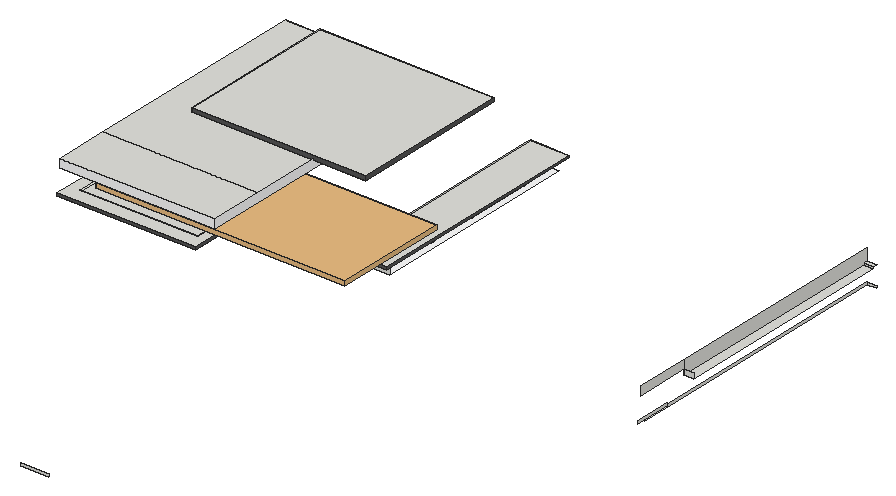
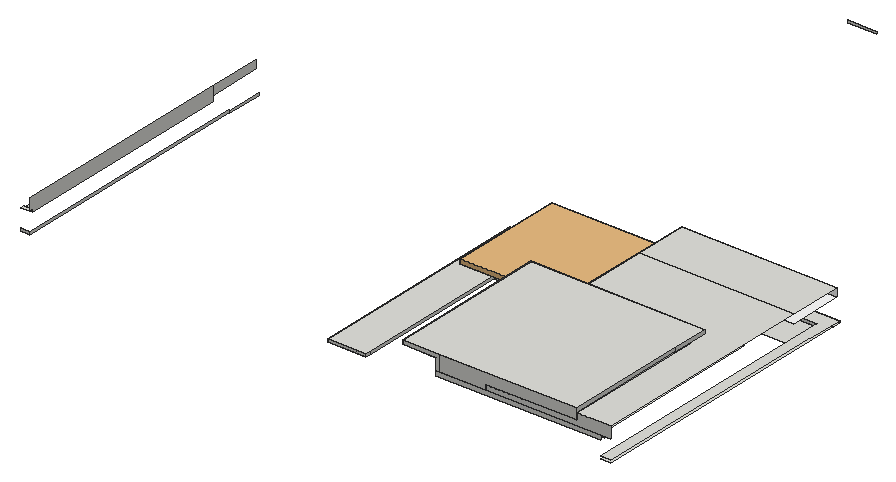
# SketchUp Ruby script. Lengths in inches.
U = 1.inch
M = Sketchup.active_model
def pt(a) = Geom::Point3d.new(a.map { |v| v * U })
def face(e, loops, mat)
  f = e.add_face(loops[0].map { |a| pt(a) })
  loops[1..].each { |l| e.add_face(l.map { |a| pt(a) }).erase! }
  f.material = f.back_material = mat if mat
  f
end
# faces: each face lists its corners as indices into pts; further lists are holes
def faces(e, pts, list, mat = nil) = list.each { |f| face(e, (f[0].is_a?(Array) ? f : [f]).map { |l| l.map { |i| pts[i] } }, mat) }
# xy, xz, yz: faces in a plane at the given z, y or x. An outline is a flat list of corners, or four numbers for a rectangle; further outlines are holes
def ring(l) = l.size == 4 ? [[l[0], l[1]], [l[2], l[1]], [l[2], l[3]], [l[0], l[3]]] : l.each_slice(2).to_a
def flat(e, list, mat, &to3) = list.each { |f| face(e, (f[0].is_a?(Array) ? f : [f]).map { |l| ring(l).map { |u, v| to3.(u, v) } }, mat) }
def xy(e, z, list, mat = nil) = flat(e, list, mat) { |x, y| [x, y, z] }
def xz(e, y, list, mat = nil) = flat(e, list, mat) { |x, z| [x, y, z] }
def yz(e, x, list, mat = nil) = flat(e, list, mat) { |y, z| [x, y, z] }
def lines(e, pts, list) = list.each { |a, b| e.add_line(pt(pts[a]), pt(pts[b])) }
# prism: a flat outline (further loops are holes) pulled along v
def prism(e, loops, v, mat = nil)
  f = face(e, loops, mat); d = Geom::Vector3d.new(v.map { |x| x * U })
  f.pushpull(f.normal.samedirection?(d) ? d.length : -d.length)
end
def box(e, o, s, mat = nil) = prism(e, [[o, [o[0] + s[0], o[1], o[2]], [o[0] + s[0], o[1] + s[1], o[2]], [o[0], o[1] + s[1], o[2]]]], [0, 0, s[2]], mat)
def at(x, y, z, deg = 0) = Geom::Transformation.translation(pt([x, y, z])) * Geom::Transformation.rotation(ORIGIN, Z_AXIS, deg.degrees)
def axes(o, x, y, z) = Geom::Transformation.new([*x, 0, *y, 0, *z, 0, *pt(o).to_a, 1])
def part(name) = M.definitions.add(name)
# library, detail: a bought-in or finely detailed component or shape, given as its bounding box
def library(name, o, s) = part(name).tap { |d| box(d.entities, o, s) }
def detail(e, o, s) = box(e.add_group.entities, o, s)
def put(e, d, t, mat = nil) = e.add_instance(d, t).tap { |i| i.material = mat if mat }
def group(e, t, mat = nil) = e.add_group.tap { |g| g.transformation = t; g.material = mat if mat }.entities
root = M.entities
M.materials.add("[Color M00]").color = [255, 255, 255]
M.materials.add("[Color M06]").color = [86, 86, 86]
c1 = library("Mesh Light\#4",[-0.5,-0.5,-0.1],[1,1,0.2])
c2 = part("Group\#24")
xy(c2.entities,0,[[203.13,95.41,201.58,95.62,200.13,96.22,198.89,97.17,197.9375,98.41,197.34,99.86,197.13,101.41,197.34,102.96,197.9375,104.41,198.89,105.65,200.13,106.61,201.58,107.21,203.13,107.41,204.6875,107.21,206.13,106.61,207.375,105.65,208.33,104.41,208.93,102.96,209.13,101.41,208.93,99.86,208.33,98.41,207.375,97.17,206.13,96.22,204.6875,95.62],[281.57,95.41,280.02,95.62,278.57,96.22,277.33,97.17,276.375,98.41,275.77,99.86,275.57,101.41,275.77,102.96,276.375,104.41,277.33,105.65,278.57,106.61,280.02,107.21,281.57,107.41,283.125,107.21,284.57,106.61,285.8125,105.65,286.77,104.41,287.37,102.96,287.57,101.41,287.37,99.86,286.77,98.41,285.8125,97.17,284.57,96.22,283.125,95.62],[350.95,95.41,349.39,95.62,347.95,96.22,346.7,97.17,345.75,98.41,345.15,99.86,344.95,101.41,345.15,102.96,345.75,104.41,346.7,105.65,347.95,106.61,349.39,107.21,350.95,107.41,352.5,107.21,353.95,106.61,355.1875,105.65,356.14,104.41,356.74,102.96,356.95,101.41,356.74,99.86,356.14,98.41,355.1875,97.17,353.95,96.22,352.5,95.62],[376,162.85,374.44,163.05,373,163.65,371.75,164.6,370.8,165.85,370.2,167.29,370,168.85,370.2,170.4,370.8,171.85,371.75,173.09,373,174.04,374.44,174.64,376,174.85,377.55,174.64,379,174.04,380.24,173.09,381.19,171.85,381.79,170.4,382,168.85,381.79,167.29,381.19,165.85,380.24,164.6,379,163.65,377.55,163.05]],"[Color M00]")
xy(c2.entities,33.4375,[[6,0,4.45,0.2,3,0.8,1.76,1.76,0.8,3,0.2,4.45,0,6,0.2,7.55,0.8,9,1.76,10.24,3,11.2,4.45,11.8,6,12,7.55,11.8,9,11.2,10.24,10.24,11.2,9,11.8,7.55,12,6,11.8,4.45,11.2,3,10.24,1.76,9,0.8,7.55,0.2],[83.125,0,81.57,0.2,80.125,0.8,78.88,1.76,77.93,3,77.33,4.45,77.125,6,77.33,7.55,77.93,9,78.88,10.24,80.125,11.2,81.57,11.8,83.125,12,84.68,11.8,86.125,11.2,87.37,10.24,88.32,9,88.92,7.55,89.125,6,88.92,4.45,88.32,3,87.37,1.76,86.125,0.8,84.68,0.2],[166.6875,0,165.13,0.2,163.6875,0.8,162.44,1.76,161.49,3,160.89,4.45,160.6875,6,160.89,7.55,161.49,9,162.44,10.24,163.6875,11.2,165.13,11.8,166.6875,12,168.24,11.8,169.6875,11.2,170.93,10.24,171.88,9,172.48,7.55,172.6875,6,172.48,4.45,171.88,3,170.93,1.76,169.6875,0.8,168.24,0.2],[166.6875,88.9375,165.13,89.14,163.6875,89.74,162.44,90.69,161.49,91.9375,160.89,93.38,160.6875,94.9375,160.89,96.49,161.49,97.9375,162.44,99.18,163.6875,100.13,165.13,100.73,166.6875,100.9375,168.24,100.73,169.6875,100.13,170.93,99.18,171.88,97.9375,172.48,96.49,172.6875,94.9375,172.48,93.38,171.88,91.9375,170.93,90.69,169.6875,89.74,168.24,89.14]],"[Color M00]")
put(c2.entities,c1,axes([191,87.42,16.72],[382.99758,0,0],[0,175.84579,0],[0,0,34.4375]))
c3 = library("Group\#23",[-0.5,-0.5,-0.1],[13,110.375,0.2])
xy(root,270.375,[[2063.54,1581.1,2275.98,1592.1],[2064.92,1592.1,2064.92,2018.36,2079.65,2018.36,2079.65,1604.38,2260.47,1604.38,2260.47,1703.22,2269.48,1703.22,2269.48,1592.1],[2269.48,1592.1,2275.98,1636.04],[2956.13,1592.1,2957.51,1636.04],[2079.65,1604.38,2260.47,1604.38,2260.47,1703.22,2256.86,1703.22,2256.86,1659.57,2079.65,1659.57],
  [2269.48,1636.04,2275.98,1728.29],[2256.86,1703.22,2269.48,1773.67]])
xy(root,274.0625,[[2063.54,1581.1,2275.98,1581.1,2275.98,1673.72,2269.48,1673.72,2269.48,1703.22,2260.47,1703.22,2260.47,1604.38,2079.65,1604.38,2079.65,2018.36,2064.92,2018.36,2064.92,1636.04,2063.54,1636.04],[2269.48,1673.72,2275.98,1728.29]])
xy(root,274.0625,[[[2275.98,1673.72,2275.98,1728.29,2459.67,1728.29,2459.67,1998.71,2500.29,1998.71,2500.29,1673.72],[2311.19,1695.77,2312.75,1695.97,2314.19,1696.57,2315.4375,1697.52,2316.39,1698.77,2316.99,1700.21,2317.19,1701.77,2316.99,1703.32,2316.39,1704.77,2315.4375,1706.01,2314.19,1706.96,2312.75,1707.5625,2311.19,1707.77,2309.64,1707.5625,2308.19,1706.96,2306.95,1706.01,2306,1704.77,2305.4,1703.32,2305.19,1701.77,2305.4,1700.21,2306,1698.77,2306.95,1697.52,2308.19,1696.57,2309.64,1695.97],[2389.63,1695.77,2391.19,1695.97,2392.63,1696.57,2393.875,1697.52,2394.83,1698.77,2395.43,1700.21,2395.63,1701.77,2395.43,1703.32,2394.83,1704.77,2393.875,1706.01,2392.63,1706.96,2391.19,1707.5625,2389.63,1707.77,2388.08,1707.5625,2386.63,1706.96,2385.39,1706.01,2384.4375,1704.77,2383.84,1703.32,2383.63,1701.77,2383.84,1700.21,2384.4375,1698.77,2385.39,1697.52,2386.63,1696.57,2388.08,1695.97],[2459.01,1695.77,2460.56,1695.97,2462.01,1696.57,2463.25,1697.52,2464.2,1698.77,2464.8,1700.21,2465.01,1701.77,2464.8,1703.32,2464.2,1704.77,2463.25,1706.01,2462.01,1706.96,2460.56,1707.5625,2459.01,1707.77,2457.45,1707.5625,2456.01,1706.96,2454.76,1706.01,2453.8125,1704.77,2453.21,1703.32,2453.01,1701.77,2453.21,1700.21,2453.8125,1698.77,2454.76,1697.52,2456.01,1696.57,2457.45,1695.97],[2484.06,1941.01,2485.61,1941.22,2487.06,1941.82,2488.3,1942.77,2489.26,1944.01,2489.86,1945.46,2490.06,1947.01,2489.86,1948.56,2489.26,1950.01,2488.3,1951.25,2487.06,1952.21,2485.61,1952.81,2484.06,1953.01,2482.51,1952.81,2481.06,1952.21,2479.82,1951.25,2478.86,1950.01,2478.26,1948.56,2478.06,1947.01,2478.26,1945.46,2478.86,1944.01,2479.82,1942.77,2481.06,1941.82,2482.51,1941.22],[2484.06,1763.2,2485.61,1763.4,2487.06,1764,2488.3,1764.96,2489.26,1766.2,2489.86,1767.65,2490.06,1769.2,2489.86,1770.75,2489.26,1772.2,2488.3,1773.44,2487.06,1774.4,2485.61,1774.99,2484.06,1775.2,2482.51,1774.99,2481.06,1774.4,2479.82,1773.44,2478.86,1772.2,2478.26,1770.75,2478.06,1769.2,2478.26,1767.65,2478.86,1766.2,2479.82,1764.96,2481.06,1764,2482.51,1763.4],[2484.06,1843.64,2485.61,1843.84,2487.06,1844.44,2488.3,1845.39,2489.26,1846.64,2489.86,1848.08,2490.06,1849.64,2489.86,1851.19,2489.26,1852.64,2488.3,1853.88,2487.06,1854.83,2485.61,1855.43,2484.06,1855.64,2482.51,1855.43,2481.06,1854.83,2479.82,1853.88,2478.86,1852.64,2478.26,1851.19,2478.06,1849.64,2478.26,1848.08,2478.86,1846.64,2479.82,1845.39,2481.06,1844.44,2482.51,1843.84]]],"[Color M00]")
xy(root,283.9375,[[2269.48,1667.47,2500.29,1673.72],[2269.48,1673.72,2269.48,1773.67,2440.84,1773.67,2440.84,2018.36,2500.29,2018.36,2500.29,1673.72]])
xy(root,287.375,[[2269.48,1667.47,2500.29,1667.47,2500.29,2018.36,2440.84,2018.36,2440.84,1773.67,2269.48,1773.67]])
xy(root,295.8125,[[2089.96,1730.8,2089.96,2011.98,2256.86,2011.98,2256.86,1851.54,2247.33,1851.54,2247.33,1730.8],[2256.86,1851.54,2327.29,2011.98]])
xy(root,299.625,[[2957.51,1667.53,2972.24,2011.98]])
xy(root,302.5625,[[2079.65,2011.98,2256.86,2018.36],[2256.86,2011.98,2327.29,2018.36],[2957.51,2011.98,2972.24,2018.36]])
xy(root,307.5,[[[2064.92,1584.22,2064.92,1667.53,2079.65,1667.53,2079.65,1636.22,2256.86,1636.22,2256.86,1829.17,2303.29,1829.17,2303.29,1584.22],[2274.75,1689.29,2276.3,1689.5,2277.75,1690.09,2278.99,1691.05,2279.95,1692.29,2280.54,1693.74,2280.75,1695.29,2280.54,1696.84,2279.95,1698.29,2278.99,1699.53,2277.75,1700.49,2276.3,1701.09,2274.75,1701.29,2273.2,1701.09,2271.75,1700.49,2270.51,1699.53,2269.55,1698.29,2268.95,1696.84,2268.75,1695.29,2268.95,1693.74,2269.55,1692.29,2270.51,1691.05,2271.75,1690.09,2273.2,1689.5],[2114.0625,1600.35,2115.61,1600.56,2117.0625,1601.16,2118.3,1602.11,2119.26,1603.35,2119.86,1604.8,2120.0625,1606.35,2119.86,1607.91,2119.26,1609.35,2118.3,1610.6,2117.0625,1611.55,2115.61,1612.15,2114.0625,1612.35,2112.51,1612.15,2111.0625,1611.55,2109.82,1610.6,2108.87,1609.35,2108.27,1607.91,2108.0625,1606.35,2108.27,1604.8,2108.87,1603.35,2109.82,1602.11,2111.0625,1601.16,2112.51,1600.56],[2191.1875,1600.35,2192.74,1600.56,2194.1875,1601.16,2195.43,1602.11,2196.38,1603.35,2196.98,1604.8,2197.1875,1606.35,2196.98,1607.91,2196.38,1609.35,2195.43,1610.6,2194.1875,1611.55,2192.74,1612.15,2191.1875,1612.35,2189.63,1612.15,2188.1875,1611.55,2186.94,1610.6,2185.99,1609.35,2185.39,1607.91,2185.1875,1606.35,2185.39,1604.8,2185.99,1603.35,2186.94,1602.11,2188.1875,1601.16,2189.63,1600.56],[2274.75,1600.35,2276.3,1600.56,2277.75,1601.16,2278.99,1602.11,2279.95,1603.35,2280.54,1604.8,2280.75,1606.35,2280.54,1607.91,2279.95,1609.35,2278.99,1610.6,2277.75,1611.55,2276.3,1612.15,2274.75,1612.35,2273.2,1612.15,2271.75,1611.55,2270.51,1610.6,2269.55,1609.35,2268.95,1607.91,2268.75,1606.35,2268.95,1604.8,2269.55,1603.35,2270.51,1602.11,2271.75,1601.16,2273.2,1600.56]]],"[Color M00]")
xy(root,310.3125,[[2117.29,1829.17,2256.86,2018.36]])
xy(root,320.75,[[2064.92,1584.22,2303.29,1667.53],[2064.92,1667.53,2303.29,1667.53,2303.29,1771.54,2117.29,1771.54,2117.29,2018.36,2064.92,2018.36],[2303.29,1771.54,2303.29,1829.17,2333.29,1829.17,2333.29,2018.36,2384.86,2018.36,2384.86,1771.54]])
xy(root,326.5,[[2117.29,1771.54,2384.86,2018.36]])
xz(root,1019,[[2456.54,283.9375,2500.29,287.375]])
xz(root,1581.1,[[2063.54,270.375,2275.98,274.0625]],"[Color M06]")
xz(root,1584.22,[[2064.92,307.5,2303.29,320.75]],"[Color M00]")
xz(root,1604.38,[[2079.65,270.375,2260.47,274.0625]])
xz(root,1636.04,[[2956.13,270.375,2957.51,274.0625]])
xz(root,1667.47,[[2269.48,283.9375,2500.29,287.375]],"[Color M06]")
xz(root,1667.53,[[2957.51,299.625,2972.24,307.5]])
xz(root,1673.72,[[2269.48,274.0625,2500.29,283.9375]])
xz(root,1703.22,[[2260.47,270.375,2269.48,274.0625]])
xz(root,1771.54,[[2117.29,320.75,2384.86,326.5]],"[Color M06]")
xz(root,1773.67,[[2269.48,283.9375,2440.84,287.375]])
xz(root,1829.17,[[2256.86,307.5,2303.29,310.3125]])
xz(root,2011.98,[[2079.65,295.8125,2256.86,302.5625],[2256.86,295.8125,2327.29,302.5625],[2957.51,299.625,2972.24,302.5625]])
xz(root,2018.36,[[2957.51,270.375,2972.24,274.0625],[2440.84,283.9375,2456.54,287.375],[2456.54,283.9375,2500.29,287.375],[2079.65,295.8125,2333.29,302.5625],[2064.92,302.5625,2064.92,320.75,2117.29,320.75,2117.29,310.3125,2256.86,310.3125,2256.86,302.5625],
  [2256.86,302.5625,2256.86,310.3125,2117.29,310.3125,2117.29,326.5,2327.29,326.5,2327.29,302.5625],[2327.29,302.5625,2327.29,326.5,2384.86,326.5,2384.86,320.75,2333.29,320.75,2333.29,302.5625]])
yz(root,2117.29,[[1801.17,310.3125,1829.17,320.75],[1829.17,310.3125,2018.36,320.75],[1771.54,320.75,1829.17,326.5],[1829.17,320.75,2018.36,326.5]])
yz(root,2256.86,[[1829.17,295.8125,2011.98,302.5625],[1829.17,302.5625,2018.36,310.3125]])
yz(root,2260.47,[[1604.38,270.375,1703.22,274.0625]])
yz(root,2269.48,[[1728.29,270.375,1728.29,274.0625,1673.72,274.0625,1673.72,283.9375,1773.67,283.9375,1773.67,270.375],[1703.22,270.375,1728.29,274.0625],[1667.47,283.9375,1773.67,287.375]])
yz(root,2275.98,[[1581.1,270.375,1728.29,274.0625]],"[Color M06]")
yz(root,2303.29,[[1584.22,307.5,1829.17,320.75]],"[Color M00]")
yz(root,2384.86,[[1771.54,320.75,2018.36,326.5]],"[Color M06]")
yz(root,2440.84,[[1773.67,283.9375,2011.98,287.375],[2011.98,283.9375,2018.36,287.375]])
yz(root,2500.29,[[1667.47,283.9375,2018.36,287.375]],"[Color M06]")
yz(root,2956.13,[[1581.1,270.375,1636.04,274.0625]])
yz(root,2957.51,[[1636.04,270.375,2018.36,274.0625],[1667.53,299.625,1667.53,320.75,2018.36,320.75,2018.36,302.5625,2011.98,302.5625,2011.98,299.625],[1584.22,307.5,1667.53,320.75]])
p = [[2311.19,1695.77,274.0625],[2309.64,1695.97,274.0625],[2309.64,1695.97,274.75],[2311.19,1695.77,274.75],[2312.75,1695.97,274.0625],[2312.75,1695.97,274.75],
  [2389.63,1695.77,274.0625],[2388.08,1695.97,274.0625],[2388.08,1695.97,274.75],[2389.63,1695.77,274.75],[2391.19,1695.97,274.0625],[2391.19,1695.97,274.75],
  [2459.01,1695.77,274.0625],[2457.45,1695.97,274.0625],[2457.45,1695.97,274.75],[2459.01,1695.77,274.75],[2460.56,1695.97,274.0625],[2460.56,1695.97,274.75],
  [2308.19,1696.57,274.0625],[2308.19,1696.57,274.75],[2314.19,1696.57,274.0625],[2314.19,1696.57,274.75],[2386.63,1696.57,274.0625],[2386.63,1696.57,274.75],
  [2392.63,1696.57,274.0625],[2392.63,1696.57,274.75],[2456.01,1696.57,274.0625],[2456.01,1696.57,274.75],[2462.01,1696.57,274.0625],[2462.01,1696.57,274.75],
  [2306.95,1697.52,274.0625],[2306.95,1697.52,274.75],[2315.4375,1697.52,274.0625],[2315.4375,1697.52,274.75],[2385.39,1697.52,274.0625],[2385.39,1697.52,274.75],
  [2393.875,1697.52,274.0625],[2393.875,1697.52,274.75],[2454.76,1697.52,274.0625],[2454.76,1697.52,274.75],[2463.25,1697.52,274.0625],[2463.25,1697.52,274.75],
  [2306,1698.77,274.0625],[2306,1698.77,274.75],[2316.39,1698.77,274.0625],[2316.39,1698.77,274.75],[2384.4375,1698.77,274.0625],[2384.4375,1698.77,274.75],
  [2394.83,1698.77,274.0625],[2394.83,1698.77,274.75],[2453.8125,1698.77,274.0625],[2453.8125,1698.77,274.75],[2464.2,1698.77,274.0625],[2464.2,1698.77,274.75],
  [2305.4,1700.21,274.0625],[2305.4,1700.21,274.75],[2316.99,1700.21,274.0625],[2316.99,1700.21,274.75],[2383.84,1700.21,274.0625],[2383.84,1700.21,274.75],
  [2395.43,1700.21,274.0625],[2395.43,1700.21,274.75],[2453.21,1700.21,274.0625],[2453.21,1700.21,274.75],[2464.8,1700.21,274.0625],[2464.8,1700.21,274.75],
  [2305.19,1701.77,274.0625],[2305.19,1701.77,274.75],[2317.19,1701.77,274.0625],[2317.19,1701.77,274.75],[2383.63,1701.77,274.0625],[2383.63,1701.77,274.75],
  [2395.63,1701.77,274.0625],[2395.63,1701.77,274.75],[2453.01,1701.77,274.0625],[2453.01,1701.77,274.75],[2465.01,1701.77,274.0625],[2465.01,1701.77,274.75],
  [2305.4,1703.32,274.0625],[2305.4,1703.32,274.75],[2316.99,1703.32,274.0625],[2316.99,1703.32,274.75],[2383.84,1703.32,274.0625],[2383.84,1703.32,274.75],
  [2395.43,1703.32,274.0625],[2395.43,1703.32,274.75],[2453.21,1703.32,274.0625],[2453.21,1703.32,274.75],[2464.8,1703.32,274.0625],[2464.8,1703.32,274.75],
  [2306,1704.77,274.0625],[2306,1704.77,274.75],[2316.39,1704.77,274.0625],[2316.39,1704.77,274.75],[2384.4375,1704.77,274.0625],[2384.4375,1704.77,274.75],
  [2394.83,1704.77,274.0625],[2394.83,1704.77,274.75],[2453.8125,1704.77,274.0625],[2453.8125,1704.77,274.75],[2464.2,1704.77,274.0625],[2464.2,1704.77,274.75],
  [2306.95,1706.01,274.0625],[2306.95,1706.01,274.75],[2315.4375,1706.01,274.0625],[2315.4375,1706.01,274.75],[2385.39,1706.01,274.0625],[2385.39,1706.01,274.75],
  [2393.875,1706.01,274.0625],[2393.875,1706.01,274.75],[2454.76,1706.01,274.0625],[2454.76,1706.01,274.75],[2463.25,1706.01,274.0625],[2463.25,1706.01,274.75],
  [2308.19,1706.96,274.0625],[2308.19,1706.96,274.75],[2314.19,1706.96,274.0625],[2314.19,1706.96,274.75],[2386.63,1706.96,274.0625],[2386.63,1706.96,274.75],
  [2392.63,1706.96,274.0625],[2392.63,1706.96,274.75],[2456.01,1706.96,274.0625],[2456.01,1706.96,274.75],[2462.01,1706.96,274.0625],[2462.01,1706.96,274.75],
  [2309.64,1707.5625,274.0625],[2309.64,1707.5625,274.75],[2312.75,1707.5625,274.0625],[2312.75,1707.5625,274.75],[2388.08,1707.5625,274.0625],[2388.08,1707.5625,274.75],
  [2391.19,1707.5625,274.0625],[2391.19,1707.5625,274.75],[2457.45,1707.5625,274.0625],[2457.45,1707.5625,274.75],[2460.56,1707.5625,274.0625],[2460.56,1707.5625,274.75],
  [2311.19,1707.77,274.0625],[2311.19,1707.77,274.75],[2389.63,1707.77,274.0625],[2389.63,1707.77,274.75],[2459.01,1707.77,274.0625],[2459.01,1707.77,274.75],
  [2484.06,1763.2,274.0625],[2482.51,1763.4,274.0625],[2482.51,1763.4,274.75],[2484.06,1763.2,274.75],[2485.61,1763.4,274.0625],[2485.61,1763.4,274.75],
  [2481.06,1764,274.0625],[2481.06,1764,274.75],[2487.06,1764,274.0625],[2487.06,1764,274.75],[2479.82,1764.96,274.0625],[2479.82,1764.96,274.75],
  [2488.3,1764.96,274.0625],[2488.3,1764.96,274.75],[2478.86,1766.2,274.0625],[2478.86,1766.2,274.75],[2489.26,1766.2,274.0625],[2489.26,1766.2,274.75],
  [2478.26,1767.65,274.0625],[2478.26,1767.65,274.75],[2489.86,1767.65,274.0625],[2489.86,1767.65,274.75],[2478.06,1769.2,274.0625],[2478.06,1769.2,274.75],
  [2490.06,1769.2,274.0625],[2490.06,1769.2,274.75],[2478.26,1770.75,274.0625],[2478.26,1770.75,274.75],[2489.86,1770.75,274.0625],[2489.86,1770.75,274.75],
  [2478.86,1772.2,274.0625],[2478.86,1772.2,274.75],[2489.26,1772.2,274.0625],[2489.26,1772.2,274.75],[2479.82,1773.44,274.0625],[2479.82,1773.44,274.75],
  [2488.3,1773.44,274.0625],[2488.3,1773.44,274.75],[2481.06,1774.4,274.0625],[2481.06,1774.4,274.75],[2487.06,1774.4,274.0625],[2487.06,1774.4,274.75],
  [2482.51,1774.99,274.0625],[2482.51,1774.99,274.75],[2485.61,1774.99,274.0625],[2485.61,1774.99,274.75],[2484.06,1775.2,274.0625],[2484.06,1775.2,274.75],
  [2484.06,1843.64,274.0625],[2482.51,1843.84,274.0625],[2482.51,1843.84,274.75],[2484.06,1843.64,274.75],[2485.61,1843.84,274.0625],[2485.61,1843.84,274.75],
  [2481.06,1844.44,274.0625],[2481.06,1844.44,274.75],[2487.06,1844.44,274.0625],[2487.06,1844.44,274.75],[2479.82,1845.39,274.0625],[2479.82,1845.39,274.75],
  [2488.3,1845.39,274.0625],[2488.3,1845.39,274.75],[2478.86,1846.64,274.0625],[2478.86,1846.64,274.75],[2489.26,1846.64,274.0625],[2489.26,1846.64,274.75],
  [2478.26,1848.08,274.0625],[2478.26,1848.08,274.75],[2489.86,1848.08,274.0625],[2489.86,1848.08,274.75],[2478.06,1849.64,274.0625],[2478.06,1849.64,274.75],
  [2490.06,1849.64,274.0625],[2490.06,1849.64,274.75],[2478.26,1851.19,274.0625],[2478.26,1851.19,274.75],[2489.86,1851.19,274.0625],[2489.86,1851.19,274.75],
  [2478.86,1852.64,274.0625],[2478.86,1852.64,274.75],[2489.26,1852.64,274.0625],[2489.26,1852.64,274.75],[2479.82,1853.88,274.0625],[2479.82,1853.88,274.75],
  [2488.3,1853.88,274.0625],[2488.3,1853.88,274.75],[2481.06,1854.83,274.0625],[2481.06,1854.83,274.75],[2487.06,1854.83,274.0625],[2487.06,1854.83,274.75],
  [2482.51,1855.43,274.0625],[2482.51,1855.43,274.75],[2485.61,1855.43,274.0625],[2485.61,1855.43,274.75],[2484.06,1855.64,274.0625],[2484.06,1855.64,274.75],
  [2484.06,1941.01,274.0625],[2482.51,1941.22,274.0625],[2482.51,1941.22,274.75],[2484.06,1941.01,274.75],[2485.61,1941.22,274.0625],[2485.61,1941.22,274.75],
  [2481.06,1941.82,274.0625],[2481.06,1941.82,274.75],[2487.06,1941.82,274.0625],[2487.06,1941.82,274.75],[2479.82,1942.77,274.0625],[2479.82,1942.77,274.75],
  [2488.3,1942.77,274.0625],[2488.3,1942.77,274.75],[2478.86,1944.01,274.0625],[2478.86,1944.01,274.75],[2489.26,1944.01,274.0625],[2489.26,1944.01,274.75],
  [2478.26,1945.46,274.0625],[2478.26,1945.46,274.75],[2489.86,1945.46,274.0625],[2489.86,1945.46,274.75],[2478.06,1947.01,274.0625],[2478.06,1947.01,274.75],
  [2490.06,1947.01,274.0625],[2490.06,1947.01,274.75],[2478.26,1948.56,274.0625],[2478.26,1948.56,274.75],[2489.86,1948.56,274.0625],[2489.86,1948.56,274.75],
  [2478.86,1950.01,274.0625],[2478.86,1950.01,274.75],[2489.26,1950.01,274.0625],[2489.26,1950.01,274.75],[2479.82,1951.25,274.0625],[2479.82,1951.25,274.75],
  [2488.3,1951.25,274.0625],[2488.3,1951.25,274.75],[2481.06,1952.21,274.0625],[2481.06,1952.21,274.75],[2487.06,1952.21,274.0625],[2487.06,1952.21,274.75],
  [2482.51,1952.81,274.0625],[2482.51,1952.81,274.75],[2485.61,1952.81,274.0625],[2485.61,1952.81,274.75],[2484.06,1953.01,274.0625],[2484.06,1953.01,274.75],
  [2114.0625,1600.35,307.5],[2112.51,1600.56,307.5],[2112.51,1600.56,308.1875],[2114.0625,1600.35,308.1875],[2115.61,1600.56,307.5],[2115.61,1600.56,308.1875],
  [2191.1875,1600.35,307.5],[2189.63,1600.56,307.5],[2189.63,1600.56,308.1875],[2191.1875,1600.35,308.1875],[2192.74,1600.56,307.5],[2192.74,1600.56,308.1875],
  [2274.75,1600.35,307.5],[2273.2,1600.56,307.5],[2273.2,1600.56,308.1875],[2274.75,1600.35,308.1875],[2276.3,1600.56,307.5],[2276.3,1600.56,308.1875],
  [2111.0625,1601.16,307.5],[2111.0625,1601.16,308.1875],[2117.0625,1601.16,307.5],[2117.0625,1601.16,308.1875],[2188.1875,1601.16,307.5],[2188.1875,1601.16,308.1875],
  [2194.1875,1601.16,307.5],[2194.1875,1601.16,308.1875],[2271.75,1601.16,307.5],[2271.75,1601.16,308.1875],[2277.75,1601.16,307.5],[2277.75,1601.16,308.1875],
  [2109.82,1602.11,307.5],[2109.82,1602.11,308.1875],[2118.3,1602.11,307.5],[2118.3,1602.11,308.1875],[2186.94,1602.11,307.5],[2186.94,1602.11,308.1875],
  [2195.43,1602.11,307.5],[2195.43,1602.11,308.1875],[2270.51,1602.11,307.5],[2270.51,1602.11,308.1875],[2278.99,1602.11,307.5],[2278.99,1602.11,308.1875],
  [2108.87,1603.35,307.5],[2108.87,1603.35,308.1875],[2119.26,1603.35,307.5],[2119.26,1603.35,308.1875],[2185.99,1603.35,307.5],[2185.99,1603.35,308.1875],
  [2196.38,1603.35,307.5],[2196.38,1603.35,308.1875],[2269.55,1603.35,307.5],[2269.55,1603.35,308.1875],[2279.95,1603.35,307.5],[2279.95,1603.35,308.1875],
  [2119.86,1604.8,307.5],[2119.86,1604.8,308.1875],[2185.39,1604.8,307.5],[2185.39,1604.8,308.1875],[2196.98,1604.8,307.5],[2196.98,1604.8,308.1875],
  [2268.95,1604.8,307.5],[2268.95,1604.8,308.1875],[2280.54,1604.8,307.5],[2280.54,1604.8,308.1875],[2120.0625,1606.35,307.5],[2120.0625,1606.35,308.1875],
  [2185.1875,1606.35,307.5],[2185.1875,1606.35,308.1875],[2197.1875,1606.35,307.5],[2197.1875,1606.35,308.1875],[2268.75,1606.35,307.5],[2268.75,1606.35,308.1875],
  [2280.75,1606.35,307.5],[2280.75,1606.35,308.1875],[2119.86,1607.91,307.5],[2119.86,1607.91,308.1875],[2185.39,1607.91,307.5],[2185.39,1607.91,308.1875],
  [2196.98,1607.91,307.5],[2196.98,1607.91,308.1875],[2268.95,1607.91,307.5],[2268.95,1607.91,308.1875],[2280.54,1607.91,307.5],[2280.54,1607.91,308.1875],
  [2119.26,1609.35,307.5],[2119.26,1609.35,308.1875],[2185.99,1609.35,307.5],[2185.99,1609.35,308.1875],[2196.38,1609.35,307.5],[2196.38,1609.35,308.1875],
  [2269.55,1609.35,307.5],[2269.55,1609.35,308.1875],[2279.95,1609.35,307.5],[2279.95,1609.35,308.1875],[2108.87,1609.35,307.5],[2109.82,1610.6,307.5],
  [2109.82,1610.6,308.1875],[2108.87,1609.35,308.1875],[2118.3,1610.6,307.5],[2118.3,1610.6,308.1875],[2186.94,1610.6,307.5],[2186.94,1610.6,308.1875],
  [2195.43,1610.6,307.5],[2195.43,1610.6,308.1875],[2270.51,1610.6,307.5],[2270.51,1610.6,308.1875],[2278.99,1610.6,307.5],[2278.99,1610.6,308.1875],
  [2111.0625,1611.55,307.5],[2111.0625,1611.55,308.1875],[2117.0625,1611.55,307.5],[2117.0625,1611.55,308.1875],[2188.1875,1611.55,307.5],[2188.1875,1611.55,308.1875],
  [2194.1875,1611.55,307.5],[2194.1875,1611.55,308.1875],[2271.75,1611.55,307.5],[2271.75,1611.55,308.1875],[2277.75,1611.55,307.5],[2277.75,1611.55,308.1875],
  [2112.51,1612.15,307.5],[2112.51,1612.15,308.1875],[2115.61,1612.15,307.5],[2115.61,1612.15,308.1875],[2189.63,1612.15,307.5],[2189.63,1612.15,308.1875],
  [2192.74,1612.15,307.5],[2192.74,1612.15,308.1875],[2273.2,1612.15,307.5],[2273.2,1612.15,308.1875],[2276.3,1612.15,307.5],[2276.3,1612.15,308.1875],
  [2114.0625,1612.35,307.5],[2114.0625,1612.35,308.1875],[2191.1875,1612.35,307.5],[2191.1875,1612.35,308.1875],[2274.75,1612.35,307.5],[2274.75,1612.35,308.1875],
  [2274.75,1689.29,307.5],[2273.2,1689.5,307.5],[2273.2,1689.5,308.1875],[2274.75,1689.29,308.1875],[2276.3,1689.5,307.5],[2276.3,1689.5,308.1875],
  [2271.75,1690.09,307.5],[2271.75,1690.09,308.1875],[2277.75,1690.09,307.5],[2277.75,1690.09,308.1875],[2270.51,1691.05,307.5],[2270.51,1691.05,308.1875],
  [2278.99,1691.05,307.5],[2278.99,1691.05,308.1875],[2269.55,1692.29,307.5],[2269.55,1692.29,308.1875],[2279.95,1692.29,307.5],[2279.95,1692.29,308.1875],
  [2268.95,1693.74,307.5],[2268.95,1693.74,308.1875],[2280.54,1693.74,307.5],[2280.54,1693.74,308.1875],[2268.75,1695.29,307.5],[2268.75,1695.29,308.1875],
  [2280.75,1695.29,307.5],[2280.75,1695.29,308.1875],[2268.95,1696.84,307.5],[2268.95,1696.84,308.1875],[2280.54,1696.84,307.5],[2280.54,1696.84,308.1875],
  [2269.55,1698.29,307.5],[2269.55,1698.29,308.1875],[2279.95,1698.29,307.5],[2279.95,1698.29,308.1875],[2270.51,1699.53,307.5],[2270.51,1699.53,308.1875],
  [2278.99,1699.53,307.5],[2278.99,1699.53,308.1875],[2271.75,1700.49,307.5],[2271.75,1700.49,308.1875],[2277.75,1700.49,307.5],[2277.75,1700.49,308.1875],
  [2273.2,1701.09,307.5],[2273.2,1701.09,308.1875],[2276.3,1701.09,307.5],[2276.3,1701.09,308.1875],[2274.75,1701.29,307.5],[2274.75,1701.29,308.1875],
  [2117.29,1801.17,310.3125],[2286.92,1801.17,310.3125],[2327.29,2011.98,302.5625],[2327.29,1829.17,302.5625],[2327.29,1851.54,295.8125],[2333.29,1851.54,295.8125],
  [2459.67,1998.71,274.0625],[2459.67,1998.71,282.1875],[2327.29,1829.17,295.8125],[2256.86,1773.67,270.375],[2256.86,1773.67,282.1875]]
faces(root,p,[[0,1,2,3],[4,0,3,5],[6,7,8,9],[10,6,9,11],[12,13,14,15],[16,12,15,17],[1,18,19,2],[20,4,5,21],
  [7,22,23,8],[24,10,11,25],[13,26,27,14],[28,16,17,29],[18,30,31,19],[32,20,21,33],[22,34,35,23],[36,24,25,37],
  [26,38,39,27],[40,28,29,41],[30,42,43,31],[44,32,33,45],[34,46,47,35],[48,36,37,49],[38,50,51,39],[52,40,41,53],
  [42,54,55,43],[56,44,45,57],[46,58,59,47],[60,48,49,61],[50,62,63,51],[64,52,53,65],[54,66,67,55],[68,56,57,69],
  [58,70,71,59],[72,60,61,73],[62,74,75,63],[76,64,65,77],[66,78,79,67],[80,68,69,81],[70,82,83,71],[84,72,73,85],
  [74,86,87,75],[88,76,77,89],[78,90,91,79],[92,80,81,93],[82,94,95,83],[96,84,85,97],[86,98,99,87],[100,88,89,101],
  [90,102,103,91],[104,92,93,105],[94,106,107,95],[108,96,97,109],[98,110,111,99],[112,100,101,113],[102,114,115,103],[116,104,105,117],
  [106,118,119,107],[120,108,109,121],[110,122,123,111],[124,112,113,125],[114,126,127,115],[128,116,117,129],[118,130,131,119],[132,120,121,133],
  [122,134,135,123],[136,124,125,137],[126,138,139,127],[138,128,129,139],[130,140,141,131],[140,132,133,141],[134,142,143,135],[142,136,137,143],
  [144,145,146,147],[148,144,147,149],[145,150,151,146],[152,148,149,153],[150,154,155,151],[156,152,153,157],[154,158,159,155],[160,156,157,161],
  [158,162,163,159],[164,160,161,165],[162,166,167,163],[168,164,165,169],[166,170,171,167],[172,168,169,173],[170,174,175,171],[176,172,173,177],
  [174,178,179,175],[180,176,177,181],[178,182,183,179],[184,180,181,185],[182,186,187,183],[188,184,185,189],[186,190,191,187],[190,188,189,191],
  [192,193,194,195],[196,192,195,197],[193,198,199,194],[200,196,197,201],[198,202,203,199],[204,200,201,205],[202,206,207,203],[208,204,205,209],
  [206,210,211,207],[212,208,209,213],[210,214,215,211],[216,212,213,217],[214,218,219,215],[220,216,217,221],[218,222,223,219],[224,220,221,225],
  [222,226,227,223],[228,224,225,229],[226,230,231,227],[232,228,229,233],[230,234,235,231],[236,232,233,237],[234,238,239,235],[238,236,237,239],
  [240,241,242,243],[244,240,243,245],[241,246,247,242],[248,244,245,249],[246,250,251,247],[252,248,249,253],[250,254,255,251],[256,252,253,257],
  [254,258,259,255],[260,256,257,261],[258,262,263,259],[264,260,261,265],[262,266,267,263],[268,264,265,269],[266,270,271,267],[272,268,269,273],
  [270,274,275,271],[276,272,273,277],[274,278,279,275],[280,276,277,281],[278,282,283,279],[284,280,281,285],[282,286,287,283],[286,284,285,287],
  [288,289,290,291],[292,288,291,293],[294,295,296,297],[298,294,297,299],[300,301,302,303],[304,300,303,305],[289,306,307,290],[308,292,293,309],
  [295,310,311,296],[312,298,299,313],[301,314,315,302],[316,304,305,317],[306,318,319,307],[320,308,309,321],[310,322,323,311],[324,312,313,325],
  [314,326,327,315],[328,316,317,329],[318,330,331,319],[332,320,321,333],[322,334,335,323],[336,324,325,337],[326,338,339,327],[340,328,329,341],
  [342,332,333,343],[334,344,345,335],[346,336,337,347],[338,348,349,339],[350,340,341,351],[352,342,343,353],[344,354,355,345],[356,346,347,357],
  [348,358,359,349],[360,350,351,361],[362,352,353,363],[354,364,365,355],[366,356,357,367],[358,368,369,359],[370,360,361,371],[372,362,363,373],
  [364,374,375,365],[376,366,367,377],[368,378,379,369],[380,370,371,381],[382,383,384,385],[386,372,373,387],[374,388,389,375],[390,376,377,391],
  [378,392,393,379],[394,380,381,395],[383,396,397,384],[398,386,387,399],[388,400,401,389],[402,390,391,403],[392,404,405,393],[406,394,395,407],
  [396,408,409,397],[410,398,399,411],[400,412,413,401],[414,402,403,415],[404,416,417,405],[418,406,407,419],[408,420,421,409],[420,410,411,421],
  [412,422,423,413],[422,414,415,423],[416,424,425,417],[424,418,419,425],[426,427,428,429],[430,426,429,431],[427,432,433,428],[434,430,431,435],
  [432,436,437,433],[438,434,435,439],[436,440,441,437],[442,438,439,443],[440,444,445,441],[446,442,443,447],[444,448,449,445],[450,446,447,451],
  [448,452,453,449],[454,450,451,455],[452,456,457,453],[458,454,455,459],[456,460,461,457],[462,458,459,463],[460,464,465,461],[466,462,463,467],
  [464,468,469,465],[470,466,467,471],[468,472,473,469],[472,470,471,473]],"[Color M00]")
lines(root,p,[[474,475],[476,477],[478,479],[480,481],[478,482],[483,484]])
put(root,c2,at(2108.0625,1600.35,274.75))
put(root,c3,at(2478.06,1843.64,274.75))
